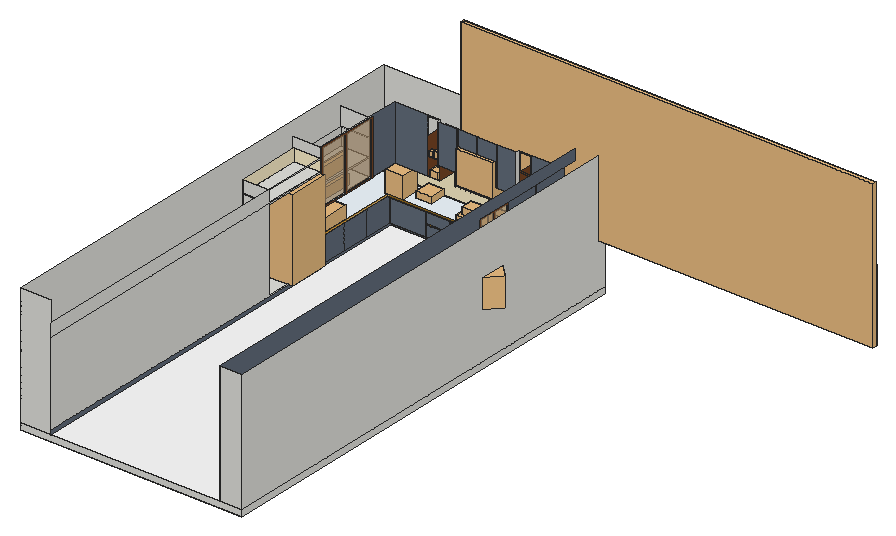
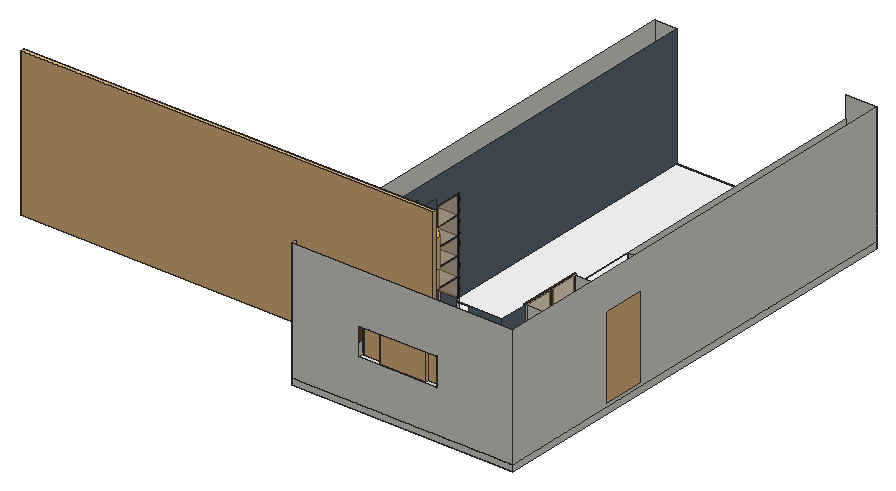
# SketchUp Ruby script. Lengths in inches.
U = 1.inch
M = Sketchup.active_model
def pt(a) = Geom::Point3d.new(a.map { |v| v * U })
def face(e, loops, mat)
  f = e.add_face(loops[0].map { |a| pt(a) })
  loops[1..].each { |l| e.add_face(l.map { |a| pt(a) }).erase! }
  f.material = f.back_material = mat if mat
  f
end
# faces: each face lists its corners as indices into pts; further lists are holes
def faces(e, pts, list, mat = nil) = list.each { |f| face(e, (f[0].is_a?(Array) ? f : [f]).map { |l| l.map { |i| pts[i] } }, mat) }
# xy, xz, yz: faces in a plane at the given z, y or x. An outline is a flat list of corners, or four numbers for a rectangle; further outlines are holes
def ring(l) = l.size == 4 ? [[l[0], l[1]], [l[2], l[1]], [l[2], l[3]], [l[0], l[3]]] : l.each_slice(2).to_a
def flat(e, list, mat, &to3) = list.each { |f| face(e, (f[0].is_a?(Array) ? f : [f]).map { |l| ring(l).map { |u, v| to3.(u, v) } }, mat) }
def xy(e, z, list, mat = nil) = flat(e, list, mat) { |x, y| [x, y, z] }
def xz(e, y, list, mat = nil) = flat(e, list, mat) { |x, z| [x, y, z] }
def yz(e, x, list, mat = nil) = flat(e, list, mat) { |y, z| [x, y, z] }
def lines(e, pts, list) = list.each { |a, b| e.add_line(pt(pts[a]), pt(pts[b])) }
# prism: a flat outline (further loops are holes) pulled along v
def prism(e, loops, v, mat = nil)
  f = face(e, loops, mat); d = Geom::Vector3d.new(v.map { |x| x * U })
  f.pushpull(f.normal.samedirection?(d) ? d.length : -d.length)
end
def box(e, o, s, mat = nil) = prism(e, [[o, [o[0] + s[0], o[1], o[2]], [o[0] + s[0], o[1] + s[1], o[2]], [o[0], o[1] + s[1], o[2]]]], [0, 0, s[2]], mat)
def at(x, y, z, deg = 0) = Geom::Transformation.translation(pt([x, y, z])) * Geom::Transformation.rotation(ORIGIN, Z_AXIS, deg.degrees)
def axes(o, x, y, z) = Geom::Transformation.new([*x, 0, *y, 0, *z, 0, *pt(o).to_a, 1])
def part(name) = M.definitions.add(name)
# library, detail: a bought-in or finely detailed component or shape, given as its bounding box
def library(name, o, s) = part(name).tap { |d| box(d.entities, o, s) }
def detail(e, o, s) = box(e.add_group.entities, o, s)
def put(e, d, t, mat = nil) = e.add_instance(d, t).tap { |i| i.material = mat if mat }
def group(e, t, mat = nil) = e.add_group.tap { |g| g.transformation = t; g.material = mat if mat }.entities
root = M.entities
M.materials.add("Generic").color = [255, 255, 255]
M.materials.add("Material__1").color = [189, 132, 57]
M.materials.add("Material__10").color = [180, 24, 1]
M.materials.add("Material__2").color = [242, 239, 230]
M.materials.add("Material__3").color = [122, 114, 11]
M.materials.add("Picture1").color = [252, 165, 11]
M.materials["Picture1"].alpha = 0.49
M.materials.add("[0093_AliceBlue]").color = [240, 248, 255]
M.materials.add("[0099_LightSteelBlue]").color = [99, 110, 124]
M.materials.add("[Color D01]").color = [255, 242, 204]
M.materials.add("[Color M00]").color = [255, 255, 255]
M.materials.add("[Color M08]").color = [30, 30, 30]
M.materials.add("[Mirror 02]").color = [198, 167, 126]
M.materials["[Mirror 02]"].alpha = 0.66
M.materials.add("[Wood Veneer 01]").color = [120, 70, 37]
M.materials.add("yellow-wall-texture-with-scratches_1249-77").color = [225, 172, 69]
M.materials["yellow-wall-texture-with-scratches_1249-77"].alpha = 0.79
c1 = library("B36CD50SNS_tradeCAD",[0,0,0],[35.84,30.35,69.65])
c2 = library("Oven",[-9.26,-22.59,0.07],[23.42,23.91,23.21])
c3 = library("Component_12",[0,0,0],[17.72,31.5,20.63])
c4 = library("CURA_RiceCooker001_fullGeometry",[-5.98,-7.38,0],[12.22,14.74,12.26])
c5 = library("jars",[-134.79,-4.32,0],[83.43,13.28,34.83])
c6 = library("Floor plant",[-5.56,-16.3125,0.81],[76.88,76.71,92.33])
c7 = library("Group\#314",[-0.26,-0.32,0],[3.72,4.79,9.78])
c8 = library("Group\#29",[55.69,-19.19,40.37],[80.08,80.05,323.81])
c9 = library("Group\#6",[0.46,121.12,-0.1],[106.94,106.94,338.14])
c10 = library("Group\#5",[151.35,137.54,-0.1],[70.51,70.14,256.45])
c11 = library("C_HOB",[0,0,0],[30.71,17.32,2.28])
c12 = library("Group\#33",[70.57,7290.35,1177],[106.36,95.58,107.8])
c13 = library("Group\#46",[141.6875,7219.59,1077.95],[111.05,77.92,100.97])
c14 = library("Group\#32",[73.8125,7223.02,1078.11],[130.55,102.07,69.6])
c15 = library("Group\#18",[51.66,7209.26,1075.25],[220.83,167.48,13.5625])
c16 = library("Group\#45",[99.22,7286.02,1075.87],[101.63,96.21,134.31])
c17 = library("Group\#47",[180.93,7251.18,1124.56],[65.88,104.93,74.66])
c18 = library("vm_v2_031",[-4.73,-4.73,0],[9.46,9.46,3.85])
c19 = library("pot",[774.13,1152.94,114],[93.39,93.39,63.05])
c20 = library("pot (1)",[31.4375,7.2,0.01],[13.32,10.03,8.54])
c21 = library("Kitchen Utensil.",[-24.86,-2.29,-26.5],[81.83,11.85,18.87])
c22 = library("Group\#305",[-29.59,-17.125,-248.78],[31.69,28.84,690.25])
c23 = library("Group1\#1",[6269.2,-3517.56,1634.27],[24.06,1609.34,28.44])
c24 = library("Group2",[6233.88,-3496.88,232.62],[78.05,1568,1448.71])
c25 = library("Group5",[6269.2,-3517.7,1199.35],[24.07,1609.51,427.52])
c26 = library("Group4",[1036.28,1705.4375,-185.71],[3176.52,4429.74,188])
c27 = library("Group3",[6262.98,-3517.7,358.33],[36.34,1611.53,831.81])
c28 = part("Component\#14")
g1 = group(c28.entities,at(-10.68,1.95,4.76),"[Color M00]")
put(g1,c22,axes([23.14,-0.3,14.16],[0,0.01831,0],[-0.00003,0,0.01479],[0.09301,0,0.00001]))
put(g1,c23,axes([140.32,80.99,-2.26],[0,-0.01299,0],[0.03988,0,0],[0,0,0.00972]))
put(g1,c24,axes([140.32,80.99,-2.26],[0,-0.01299,0],[0.03988,0,0],[0,0,0.00972]))
put(g1,c25,axes([140.32,80.99,-2.26],[0,-0.01299,0],[0.03988,0,0],[0,0,0.00972]))
put(g1,c26,axes([453.5,-0.87,-26.375],[-0.10583,0,-0.00001],[-0.00003,0,0.01683],[0,0.02083,0]))
put(g1,c27,axes([140.32,80.99,-2.26],[0,-0.01299,0],[0.03988,0,0],[0,0,0.00972]))
c29 = library("Sliding+Window+Aluminium",[0,0,0],[47.24,2.91,49.21])
c30 = part("KITCHEN WINDOW")
put(c30.entities,c28,axes([5.29,0,-9.32],[0,1.21595,0],[-1,0,0],[0,0,1.95846]),"[Color M00]")
put(c30.entities,c29,axes([2.91,0,0],[0,0.95003,0],[-1,0,0],[0,0,0.57302]))
c31 = library("Untitled (21)",[34.56,5.78,0],[33.51,33.52,23.62])
c32 = library("Group\#261",[-433.81,-170.65,316.14],[99.3,128.23,183.55])
c33 = library("Group\#262",[-328.66,-188.67,316.12],[151.64,146.26,158.64])
c34 = library("Food+jars (1)",[-3.15,-4.1,0],[15.4,16.05,11.47])
c35 = library("Group\#16",[-397.46,82.38,-0.11],[62.88,62.86,260])
c36 = library("Group\#14",[-282.65,82.375,-0.11],[62.85,62.875,260.02])
c37 = library("Group\#15",[222.96,189.98,-0.44],[259.48,39.25,337.49])
c38 = library("Group\#30",[41.52,-158.49,40.25],[95.93,90.14,172.87])
c39 = library("Group\#13",[-504.125,120.57,-0.1],[108.2,108.21,338.13])
c40 = library("Group\#12",[-376.9,120.94,-0.1],[107.79,107.8,326.37])
c41 = library("Group\#11",[-254.81,120.48,-0.6],[108.21,108.21,334.5])
c42 = library("Group\#10",[-133.01,121.19,-0.1],[106.95,106.95,324.89])
c43 = library("Group\#27",[-266.02,-201.27,40.23],[225.02,228.69,89.38])
c44 = library("Group\#28",[-78.56,-74.98,40.25],[131.28,107.59,245.3125])
c45 = library("Group\#31",[-60.55,-181.2,40.41],[105.85,106.35,65.49])
c46 = library("Group\#34",[253.59,42.68,151.97],[53.13,53.13,100.94])
c47 = library("Group\#35",[281.12,-5,151.97],[53.13,53.13,100.92])
c48 = library("Group\#36",[308.75,-52.85,151.97],[53.125,53.13,100.94])
c49 = library("Group\#37",[336.19,-100.38,151.98],[53.13,53.13,100.93])
c50 = library("Group\#38",[363.79,-148.1875,151.98],[53.13,53.13,100.93])
c51 = library("Group\#39",[253.59,42.68,30.7],[53.13,53.13,100.93])
c52 = library("Group\#40",[281.12,-5,30.7],[53.13,53.13,100.91])
c53 = library("Group\#41",[308.75,-52.85,30.7],[53.125,53.13,100.94])
c54 = library("Group\#42",[336.19,-100.38,30.7],[53.13,53.13,100.91])
c55 = library("Group\#43",[363.79,-148.1875,30.7],[53.13,53.13,100.93])
c56 = library("Group\#44",[212.54,-198.04,-0.24],[263.36,352.65,298.47])
c57 = part("KITCHEN+ITEMS+(1) (1)")
put(c57.entities,c35,at(0,0,0))
put(c57.entities,c36,at(0,0,0))
put(c57.entities,c37,at(0,0,0))
put(c57.entities,c38,at(0,0,-41.3))
put(c57.entities,c39,at(0,0,0))
put(c57.entities,c40,at(0,0,0))
put(c57.entities,c41,at(0,0,0))
put(c57.entities,c42,at(0,0,0))
put(c57.entities,c9,at(0,0,0))
put(c57.entities,c10,at(0,0,0))
put(c57.entities,c43,at(0,0,-41.3))
put(c57.entities,c44,at(0,0,-41.3))
put(c57.entities,c45,at(0,0,-41.3))
put(c57.entities,c46,at(0,0,0))
put(c57.entities,c47,at(0,0,0))
put(c57.entities,c48,at(0,0,0))
put(c57.entities,c49,at(0,0,0))
put(c57.entities,c50,at(0,0,0))
put(c57.entities,c51,at(0,0,0))
put(c57.entities,c52,at(0,0,0))
put(c57.entities,c53,at(0,0,0))
put(c57.entities,c54,at(0,0,0))
put(c57.entities,c55,at(0,0,0))
put(c57.entities,c56,at(0,0,0))
put(c57.entities,c8,at(0,0,-41.3))
c58 = library("Group\#260",[0,0,0],[30.82,7.02,10])
c59 = library("PV977NSS_GEProfile",[-17.9375,-27.5625,-0.25],[35.95,27.64,32.08])
c60 = library("Group\#252",[395.59,-144.07,554.28],[103.86,103.86,170.6])
c61 = library("Group\#253",[278.63,-144.07,554.28],[103.86,103.86,170.6])
c62 = library("Group\#254",[163.08,-144.02,554.28],[103.75,103.76,170.6])
c63 = library("Group\#120",[0,0,0],[7.01,7.02,8.25])
c64 = library("Group\#121",[0,0,0],[7,7.02,8.25])
c65 = library("KITCHEN+ITEMS+(3)",[-2.27,-9.02,0],[4.03,10.9,5.45])
xy(root,-6,[[0,0,220,450.125]])
xy(root,0,[[0,0,30,0,30,335,28.4375,335,28.4375,423.125,198,423.125,198,0,220,0,220,450.125,0,450.125]])
xy(root,0,[[30,0,198,0,198,423.125,28.4375,423.125,28.4375,335,30,335]],"Generic")
xy(root,1.01,[[198,271.14,218.5625,296.01]])
xy(root,4,[[28.4375,335,30,363.375],[198,354.34,198.25,354.64],[28.4375,363.375,29.75,363.68],[28.4375,363.68,30,391.75],[198,387.08,198.25,387.38],
  [28.4375,391.75,29.75,392.05],[28.4375,392.05,30,420.125],[28.4375,420.125,30,423.125],[30,420.125,30,423.125,198,423.125,198,420.125,162.3,420.125,162.3,420.375,162,420.375,162,420.125,148.11,420.125,148.11,420.375,147.8125,420.375,147.8125,420.125,138.3,420.125,138.3,420.375,138,420.375,138,420.125,90.3,420.125,90.3,420.375,90,420.375,90,420.125,66.3,420.125,66.3,420.375,66,420.375,66,420.125],[30,423.125,198,444.125]])
xy(root,4.56,[[4.125,270.68,30,334.44]])
xy(root,14.83,[[66.3,420.125,90,420.375],[90.3,420.125,138,420.375]])
xy(root,16,[[66.3,420.125,90,420.375],[90.3,420.125,138,420.375]])
xy(root,16.55,[[198,354.64,198.25,387.08],[198,387.38,198.25,405.02]])
xy(root,17.8,[[198,354.64,198.25,387.08],[198,387.38,198.25,405.02]])
xy(root,17.91,[[198,271.14,218.5625,296.01]])
xy(root,19.16,[[198,271.14,218.5625,296.01]])
xy(root,19.5,[[6.85,342.875,28.23,368.375]])
xy(root,20.5625,[[198,297.58,219,321.38]])
xy(root,23.49,[[90.3,420.125,138,420.375]])
xy(root,24.79,[[90.3,420.125,138,420.375]])
xy(root,28,[[198,354.34,198.25,354.64],[29.75,363.375,30,363.68],[198,387.08,198.25,387.38],[29.75,391.75,30,392.05],[30,418.125,30,420.125,66,420.125,66,420.375,66.3,420.375,66.3,420.125,90,420.125,90,420.375,90.3,420.375,90.3,420.125,138,420.125,138,420.375,138.3,420.375,138.3,420.125,147.8125,420.125,147.8125,420.375,148.11,420.375,148.11,420.125,162,420.125,162,420.375,162.3,420.375,162.3,420.125,198,420.125,198,418.125],
  [30,420.125,30,444.125,198,444.125,198,420.125,162.3,420.125,162.3,420.375,162,420.375,162,420.125,148.11,420.125,148.11,420.375,147.8125,420.375,147.8125,420.125,138.3,420.125,138.3,420.375,138,420.375,138,420.125,90.3,420.125,90.3,420.375,90,420.375,90,420.125,66.3,420.125,66.3,420.375,66,420.375,66,420.125],[30,444.125,198,445.125]])
xy(root,30,[[30,444.125,198,445.125]])
xy(root,30,[[[198,321.9,217,321.9,217,444.125,4.125,444.125,4.125,335,30,335,30,418.125,198,418.125],[6.85,342.875,28.23,368.375]]],"[0093_AliceBlue]")
xy(root,36.5625,[[198,271.14,218.5625,296.01]])
xy(root,37.3125,[[198,271.14,218.5625,296.01]])
xy(root,41.71,[[75.375,444.125,76.375,444.125,76.375,445.125],[75.375,444.125,76.375,445.125,76.375,444.125,153.5625,444.125,153.5625,450.125,75.375,450.125]])
xy(root,45.21,[[198,297.58,219,321.38]])
xy(root,47.25,[[198,297.58,219,321.38]])
xy(root,54,[[198,321.9,198,356.64,198.3,356.64,198.3,356.94,197.6875,356.94,197.6875,408.75,198,408.75,198,426.125,217,426.125,217,321.9],[4.125,335,4.125,444.125,75.375,444.125,75.375,426.125,30,426.125,30,335],[153.5625,426.125,217,444.125]],"[0099_LightSteelBlue]")
xy(root,54.47,[[198,271.14,218.5625,296.01]])
xy(root,54.54,[[154.0625,426.125,165.5625,448.75]],"[Wood Veneer 01]")
xy(root,54.6,[[63.375,426.125,74.78,448.75]],"[Wood Veneer 01]")
xy(root,54.64,[[198,322.54,215.4375,356]])
xy(root,54.89,[[197.6875,357.27,219.8125,407.18]],"[Wood Veneer 01]")
xy(root,54.99,[[0.8125,335.99,30,396.27]])
xy(root,55.47,[[198,271.14,218.5625,296.01]])
xy(root,69.8125,[[75.375,422.75,75.375,450.125,153.5625,450.125,153.5625,422.75,134.32,422.75,134.32,423.05,134.02,423.05,134.02,422.75,114.77,422.75,114.77,423.05,114.47,423.05,114.47,422.75,95.22,422.75,95.22,423.05,94.92,423.05,94.92,422.75]],"[0099_LightSteelBlue]")
xy(root,70.6,[[197.6875,357.27,219.8125,407.18]],"[Wood Veneer 01]")
xy(root,71.24,[[197.6875,356.94,198,391.08],[197.6875,391.08,198,391.38],[197.6875,391.38,198,408.75]])
xy(root,71.51,[[154.0625,426.125,155.1875,448.75],[155.1875,426.125,165.5625,448.75]],"[Wood Veneer 01]")
xy(root,71.53,[[0.8125,335.99,28.4375,396.27]])
xy(root,72.2,[[154.0625,426.125,165.5625,448.75]])
xy(root,72.2,[[63.375,426.125,74.78,448.75]],"[Wood Veneer 01]")
xy(root,72.37,[[198,322.54,215.4375,339.38],[198,339.38,215.4375,339.91],[198,339.91,215.4375,356]])
xy(root,72.53,[[0.8125,335.99,28.4375,396.27]])
xy(root,72.82,[[63.375,426.125,74.78,448.75]])
xy(root,72.84,[[198,322.54,215.4375,356]])
xy(root,72.93,[[198,271.14,218.5625,296.01]])
xy(root,73.62,[[198,271.14,218.5625,296.01]])
xy(root,76.02,[[198,297.58,219,321.38]])
xy(root,85.63,[[4.125,270.68,30,334.44]])
xy(root,86.74,[[4.125,270.68,30,334.44]])
xz(root,0,[[0,-6,220,0],[0,0,30,120],[198,0,220,120]])
xz(root,270.68,[[4.125,4.56,30,85.63],[4.125,86.74,30,98.53]])
xz(root,271.14,[[198,1.01,218.5625,17.91],[198,19.16,218.5625,36.5625],[198,37.3125,218.5625,54.47],[198,55.47,218.5625,72.93],[198,73.62,218.5625,91.77]])
xz(root,296.01,[[198,1.01,218.5625,17.91],[198,19.16,218.5625,36.5625],[198,37.3125,218.5625,54.47],[198,55.47,218.5625,72.93],[198,73.62,218.5625,91.77]])
xz(root,297.58,[[198,20.5625,219,45.21],[198,47.25,219,76.02]])
xz(root,321.38,[[198,20.5625,219,28],[198,28,219,30],[198,30,219,45.21],[198,47.25,219,54],[198,54,219,76.02]])
xz(root,321.9,[[198,30,217,54]])
xz(root,322.54,[[198,54.64,215.4375,72.37],[198,72.84,215.4375,90.38]])
xz(root,334.44,[[4.125,4.56,30,85.63]])
xz(root,334.44,[[4.125,86.74,30,98.53]],"[Color D01]")
xz(root,335,[[28.4375,0,30,4],[4.125,30,30,54]])
xz(root,335.99,[[0.8125,54.99,0.8125,71.53,28.4375,71.53,28.4375,72.53,0.8125,72.53,0.8125,86.1875,30,86.1875,30,54.99],[0.8125,86.1875,0.8125,89.07,28.4375,89.07,28.4375,90.07,0.8125,90.07,0.8125,107.6,30,107.6,30,86.1875]])
xz(root,342.875,[[6.85,19.5,28.23,30]])
xz(root,354.34,[[198,4,198.25,28]])
xz(root,354.64,[[198,4,198.25,16.55],[198,16.55,198.25,17.8],[198,17.8,198.25,28]])
xz(root,356,[[198,54.64,215.4375,72.37],[198,72.84,215.4375,90.38]])
xz(root,356.64,[[198,54,198.3,108.59]])
xz(root,356.94,[[197.6875,54,198.3,54,198.3,108.59,198,108.59,198,71.24,197.6875,71.24]])
xz(root,357.27,[[197.6875,54.89,219.8125,70.6]])
xz(root,363.375,[[29.75,4,30,28]])
xz(root,363.68,[[29.75,4,30,28]])
xz(root,368.375,[[6.85,19.5,28.23,30]])
xz(root,387.08,[[198,4,198.25,16.55],[198,16.55,198.25,17.8],[198,17.8,198.25,28]])
xz(root,387.38,[[198,4,198.25,16.55],[198,16.55,198.25,17.8],[198,17.8,198.25,28]])
xz(root,391.75,[[29.75,4,30,28]])
xz(root,392.05,[[29.75,4,30,28]])
xz(root,396.27,[[0.8125,54.99,30,54.99,30,107.6,0.8125,107.6,0.8125,90.07,28.4375,90.07,28.4375,89.07,0.8125,89.07,0.8125,72.53,28.4375,72.53,28.4375,71.53,0.8125,71.53]])
xz(root,405.02,[[198,16.55,198.25,17.8]])
xz(root,407.18,[[197.6875,54.89,219.8125,70.6]],"[Wood Veneer 01]")
xz(root,408.75,[[197.6875,54,198,71.24]])
xz(root,418.125,[[30,28,198,30]],"Picture1")
xz(root,420.125,[[30,4,66,28],[66.3,4,90,14.83],[90.3,4,138,14.83],[138.3,4,147.8125,28],[148.11,4,162,28],
  [162.3,4,198,28],[66.3,16,90,28],[90.3,16,138,23.49],[90.3,24.79,138,28]],"[0099_LightSteelBlue]")
xz(root,420.375,[[66,4,66.3,28],[90,4,90.3,28],[138,4,138.3,28],[147.8125,4,148.11,28],[162,4,162.3,28]])
xz(root,420.375,[[66.3,14.83,90,16],[90.3,14.83,138,16],[90.3,23.49,138,24.79]],"Picture1")
xz(root,422.75,[[75.375,69.8125,94.92,108.59],[95.22,69.8125,114.47,108.59],[114.77,69.8125,134.02,108.59],[134.32,69.8125,153.5625,108.59]],"[0099_LightSteelBlue]")
xz(root,423.05,[[94.92,69.8125,95.22,108.59],[114.47,69.8125,114.77,108.59],[134.02,69.8125,134.32,108.59]])
xz(root,423.125,[[28.4375,0,198,4]],"[0099_LightSteelBlue]")
xz(root,426.125,[[30,54,62.83,108.59],[166.25,54,198,108.59]],"[0099_LightSteelBlue]")
xz(root,426.125,[[[62.83,54,75.375,108.59],[63.375,54.6,74.78,107.92]],[[153.5625,54,166.25,108.59],[154.0625,90.4,165.5625,108.12],[154.0625,72.2,165.5625,89.71],[154.0625,54.54,165.5625,71.51]],[63.375,72.2,74.78,72.82]],"[Wood Veneer 01]")
xz(root,444.125,[[30,4,198,28],[30,28,198,30]])
xz(root,444.125,[[4.125,30,217,30,217,54,153.5625,54,153.5625,41.71,75.375,41.71,75.375,54,4.125,54]],"[Color D01]")
xz(root,445.125,[[30,28,198,30]])
xz(root,448.75,[[154.0625,54.54,165.5625,71.51],[63.375,54.6,74.78,72.2],[154.0625,72.2,165.5625,89.71],[63.375,72.82,74.78,90.4]],"[Wood Veneer 01]")
xz(root,450.125,[[0,-6,220,0],[[0,0,220,120],[75.375,41.71,153.5625,69.8125]]])
yz(root,0,[[0,-6,450.125,0],[0,0,450.125,120]])
yz(root,0.8125,[[335.99,54.99,396.27,71.53],[335.99,72.53,396.27,89.07]])
yz(root,4.125,[[270.68,4.56,334.44,85.63]])
yz(root,4.125,[[335,30,444.125,54],[270.68,86.74,334.44,98.53]],"[Color D01]")
yz(root,6.85,[[342.875,19.5,368.375,30]])
yz(root,28.23,[[342.875,19.5,368.375,30]])
yz(root,28.4375,[[335.99,71.53,396.27,72.53]])
yz(root,28.4375,[[335,0,423.125,4]],"[0099_LightSteelBlue]")
yz(root,29.75,[[363.375,4,363.68,28],[391.75,4,392.05,28]])
yz(root,30,[[[0,4,335,86.1875],[270.68,4.56,334.44,85.63]],[420.125,4,444.125,28],[444.125,28,445.125,30],[[335,54,397.27,108.59],[335.99,54.99,396.27,107.6]],[[0,86.1875,335,99.09],[270.68,86.74,334.44,98.53]]])
yz(root,30,[[335,28,418.125,30]],"Picture1")
yz(root,30,[[0,0,335,4],[335,4,363.375,28],[363.68,4,391.75,28],[392.05,4,420.125,28],[397.27,54,426.125,108.59]],"[0099_LightSteelBlue]")
yz(root,63.375,[[426.125,54.6,448.75,72.2],[426.125,72.82,448.75,90.4]],"[Wood Veneer 01]")
yz(root,66,[[420.125,4,420.375,28]])
yz(root,66.3,[[420.125,4,420.375,14.83],[420.125,16,420.375,28]])
yz(root,74.78,[[426.125,54.6,448.75,72.2],[426.125,72.82,448.75,90.4]],"[Wood Veneer 01]")
yz(root,75.375,[[444.125,41.71,450.125,54],[422.75,69.8125,426.125,108.59]])
yz(root,75.375,[[426.125,54,450.125,69.8125]],"[Wood Veneer 01]")
yz(root,90,[[420.125,4,420.375,14.83],[420.125,16,420.375,28]])
yz(root,90.3,[[420.125,4,420.375,14.83],[420.125,16,420.375,23.49],[420.125,24.79,420.375,28]])
yz(root,94.92,[[422.75,69.8125,423.05,108.59]])
yz(root,95.22,[[422.75,69.8125,423.05,108.59]])
yz(root,114.47,[[422.75,69.8125,423.05,108.59]])
yz(root,114.77,[[422.75,69.8125,423.05,108.59]])
yz(root,134.02,[[422.75,69.8125,423.05,108.59]])
yz(root,134.32,[[422.75,69.8125,423.05,108.59]])
yz(root,138,[[420.125,4,420.375,14.83],[420.125,16,420.375,23.49],[420.125,24.79,420.375,28]])
yz(root,138.3,[[420.125,4,420.375,28]])
yz(root,147.8125,[[420.125,4,420.375,28]])
yz(root,148.11,[[420.125,4,420.375,28]])
yz(root,153.5625,[[444.125,41.71,450.125,54],[422.75,69.8125,426.125,108.59]])
yz(root,153.5625,[[426.125,54,450.125,69.8125]],"[Wood Veneer 01]")
yz(root,154.0625,[[426.125,54.54,448.75,71.51],[426.125,72.2,448.75,89.71]],"[Wood Veneer 01]")
yz(root,162,[[420.125,4,420.375,28]])
yz(root,162.3,[[420.125,4,420.375,28]])
yz(root,165.5625,[[426.125,54.54,448.75,71.51],[426.125,72.2,448.75,89.71]],"[Wood Veneer 01]")
yz(root,197.6875,[[[356.94,54,408.75,71.24],[357.27,54.89,407.18,70.6]]],"[Wood Veneer 01]")
yz(root,198,[[354.34,4,354.64,28],[387.08,4,387.38,16.55],[420.125,4,444.125,28],[387.08,16.55,387.38,17.8],[387.08,17.8,387.38,28],
  [271.14,17.91,296.01,19.16],[[297.0625,20.04,321.9,45.73],[297.58,20.5625,321.38,45.21]],[444.125,28,445.125,30],[271.14,36.5625,296.01,37.3125],[297.0625,45.73,321.9,46.73],
  [[297.0625,46.73,321.9,76.54],[297.58,47.25,321.38,76.02]],[[321.9,54,356.64,108.59],[322.54,54.64,356,72.37],[322.54,72.84,356,90.38],[322.54,91.04,356,107.95]],[271.14,54.47,296.01,55.47],[391.08,71.24,391.38,108.59],[271.14,72.93,296.01,73.62]])
yz(root,198,[[321.9,28,418.125,30]],"Picture1")
yz(root,198,[[0,0,0,120,444.125,120,444.125,108.59,321.9,108.59,321.9,100.71,297.04,100.71,297.04,100.15,297.0625,92.9375,268.76,92.9375,268.46,0],[297.0625,0,321.9,20.04],[321.9,0,423.125,4],[321.9,4,354.34,28],[354.64,4,387.08,16.55],
  [387.38,4,387.38,16.55,405.02,16.55,405.02,17.8,387.38,17.8,387.38,28,420.125,28,420.125,4],[354.64,17.8,387.08,28],[408.75,54,408.75,71.24,391.38,71.24,391.38,108.59,426.125,108.59,426.125,54],[356.94,71.24,391.08,108.59],[297.0625,76.54,297.0625,92.9375,297.04,100.15,321.9,100.15,321.9,76.54]],"[0099_LightSteelBlue]")
yz(root,198,[[[268.46,0,268.76,92.9375,297.0625,92.9375,297.0625,0],[271.14,1.01,296.01,91.77]]],"[Color M08]")
yz(root,198,[[271.14,1.01,296.01,17.91],[271.14,19.16,296.01,36.5625],[271.14,37.3125,296.01,54.47],[271.14,55.47,296.01,72.93],[271.14,73.62,296.01,91.77]],"[Mirror 02]")
yz(root,198,[[354.64,16.55,387.08,17.8]],"yellow-wall-texture-with-scratches_1249-77")
yz(root,198.25,[[354.34,4,354.64,28],[387.08,4,387.38,28],[354.64,16.55,387.08,17.8]])
yz(root,198.25,[[387.38,16.55,405.02,17.8]],"yellow-wall-texture-with-scratches_1249-77")
yz(root,198.3,[[356.64,54,356.94,108.59]])
yz(root,215.4375,[[322.54,54.64,356,72.37],[322.54,72.84,356,90.38]])
yz(root,217,[[321.9,30,444.125,54]],"[Color D01]")
yz(root,218.5625,[[271.14,1.01,296.01,17.91],[271.14,19.16,296.01,36.5625],[271.14,37.3125,296.01,54.47],[271.14,55.47,296.01,72.93],[271.14,73.62,296.01,91.77]])
yz(root,219,[[297.58,20.5625,321.38,45.21],[297.58,47.25,321.38,76.02]])
yz(root,219.8125,[[357.27,54.89,407.18,70.6]],"[Wood Veneer 01]")
yz(root,220,[[0,-6,450.125,0],[0,0,450.125,120]])
p = [[207.95,274.79,0],[198,296.01,0],[198,298.35,0],[198,298.35,-2.34],[153.53,444.36,53.89],[167.85,444.125,54],
  [153.5625,444.125,54],[153.53,444.125,54],[153.5625,444.125,69.8125]]
lines(root,p,[[0,1],[2,3],[4,5],[6,7],[7,8]])
put(root,c1,axes([34.86,293.64,4.56],[0,1.1386,0],[-1.16,0,0],[0,0,1.16]))
put(root,c2,axes([218.31,312.19,20.46],[0,-0.99882,0],[1,0,0],[0,0,1.06311]))
put(root,c3,axes([7.16,342.79,20.83],[1.19,0,0],[0,0.8122,0],[0,0,1]))
put(root,c4,at(206.73,344.04,30,180))
put(root,c5,axes([217.02,426.57,30],[0.2077,0,0],[0,0.2077,0],[0,0,0.2077]))
put(root,c6,axes([28.27,421.88,29.8125],[0.23,0,0],[0,0.23,0],[0,0,0.23]))
put(root,c7,at(171.86,428.97,30,180))
g2 = group(root,at(172.19,425.85,30))
put(g2,c8,axes([6.11,1.19,-1.42],[0.0352,0,0],[0,0.0352,0],[0,0,0.0352]))
put(g2,c9,axes([-0.02,-4.26,0.03],[0.0352,0,0],[0,0.0352,0],[0,0,0.0352]))
put(g2,c10,axes([-0.02,-4.26,0.03],[0.0352,0,0],[0,0.0352,0],[0,0,0.0352]))
put(root,c11,axes([94.87,420.74,30],[1.308,0,0],[0,1.308,0],[0,0,1.308]))
g3 = group(root,at(200.95,354.48,30))
g4 = group(g3,at(-2.96,-412.37,-61.43),"Material__1")
detail(g4,[10.46,416.25,61.43],[3.24,3.12,3.51])
put(g3,c12,axes([-2.96,-412.37,-61.43],[0.0572,0,0],[0,0.0572,0],[0,0,0.0572]))
put(g3,c13,axes([-2.96,-412.37,-61.43],[0.0572,0,0],[0,0.0572,0],[0,0,0.0572]),"Material__1")
put(g3,c14,axes([-2.96,-412.37,-61.43],[0.0572,0,0],[0,0.0572,0],[0,0,0.0572]),"Material__3")
put(g3,c15,axes([-2.96,-412.37,-61.43],[0.0572,0,0],[0,0.0572,0],[0,0,0.0572]),"Material__2")
put(g3,c16,axes([-2.96,-412.37,-61.43],[0.0572,0,0],[0,0.0572,0],[0,0,0.0572]))
put(g3,c17,axes([-2.96,-412.37,-61.43],[0.0572,0,0],[0,0.0572,0],[0,0,0.0572]),"Material__10")
put(root,c18,axes([58,435.27,30],[1.62,0,0],[0,1.62,0],[0,0,1.62]))
put(root,c19,axes([2.99,285.06,17.98],[0.1218,0,0],[0,0.1218,0],[0,0,0.1218]))
put(root,c20,at(89.34,420.95,32.97))
put(root,c21,axes([215.49,392.78,56.8125],[0,0.51691,0],[-0.66,0,0],[0,0,0.66]))
put(root,c30,at(88.36,448.48,41.71,-90),"[Color D01]")
put(root,c31,axes([156.44,330.09,47.32],[0.70957,-0.70463,0],[0.70463,0.70957,0],[0,0,1.21]))
g5 = group(root,at(197.53,321.9,54),"[Wood Veneer 01]")
xy(g5,0,[[0,0,0.9375,34.74]])
xy(g5,0.64,[[0,0.64,0.47,17.48],[0.47,0.64,0.9375,17.48],[0,18.01,0.47,34.1],[0.47,18.01,0.9375,34.1]])
xy(g5,53.95,[[0,0.64,0.47,17.48],[0.47,0.64,0.9375,17.48],[0,18.01,0.47,34.1],[0.47,18.01,0.9375,34.1]])
xy(g5,54.59,[[0,0,0.9375,34.74]])
xz(g5,0,[[0,0,0.9375,22.54],[0,22.54,0.9375,54.59]])
xz(g5,0.64,[[0,0.64,0.47,53.95],[0.47,0.64,0.9375,53.95]])
xz(g5,17.48,[[0,0.64,0.47,53.95],[0.47,0.64,0.9375,53.95]])
xz(g5,18.01,[[0,0.64,0.47,53.95],[0.47,0.64,0.9375,53.95]])
xz(g5,34.1,[[0,0.64,0.47,53.95],[0.47,0.64,0.9375,53.95]])
xz(g5,34.74,[[0,0,0.9375,54.59]])
yz(g5,0,[[[0,0,34.74,54.59],[0.64,0.64,17.48,53.95],[18.01,0.64,34.1,53.95]]])
yz(g5,0.47,[[0.64,0.64,17.48,53.95],[18.01,0.64,34.1,53.95]],"[Mirror 02]")
yz(g5,0.9375,[[[0,0,34.74,54.59],[0.64,0.64,17.48,53.95],[18.01,0.64,34.1,53.95]]])
g6 = group(root,at(30,335,54),"[Wood Veneer 01]")
yz(g6,0.66,[[0.99,0.99,28.84,53.6],[30.15,0.99,61.27,53.6]],"[Mirror 02]")
g7 = group(g6,at(0,0,0))
xy(g7,0,[[0,0,1.3125,62.27]])
xy(g7,0.99,[[0,0.99,1.3125,28.84],[0,30.15,1.3125,61.27]])
xy(g7,53.6,[[0,0.99,1.3125,28.84],[0,28.84,1.3125,30.15],[0,30.15,1.3125,61.27]])
xy(g7,54.59,[[0,0,1.3125,62.27]])
xz(g7,0,[[0,0,1.3125,32.1875],[0,32.1875,1.3125,54.59]])
xz(g7,0.99,[[0,0.99,1.3125,32.1875],[0,32.1875,1.3125,53.6]])
xz(g7,28.84,[[0,0.99,1.3125,53.6]])
xz(g7,30.15,[[0,0.99,1.3125,53.6]])
xz(g7,61.27,[[0,0.99,1.3125,53.6]])
xz(g7,62.27,[[0,0,1.3125,54.59]])
yz(g7,0,[[[0,0,62.27,54.59],[30.15,0.99,61.27,53.6],[0.99,0.99,28.84,53.6]]])
yz(g7,1.3125,[[[0,0,62.27,54.59],[30.15,0.99,61.27,53.6],[0.99,0.99,28.84,53.6]]])
g8 = group(root,at(164.85,432.27,54.54))
put(g8,c32,axes([-18.22,-7.92,-13.28],[-0.042,0,0],[0,-0.042,0],[0,0,0.042]))
put(g8,c33,axes([-18.22,-7.92,-13.28],[-0.042,0,0],[0,-0.042,0],[0,0,0.042]))
put(root,c34,axes([71.33,432.1,54.6],[-0.5005,0,0],[0,-0.5005,0],[0,0,0.5005]))
put(root,c57,axes([204.57,385.96,54.92],[0,-0.04208,0],[0.03102,0,0],[0,0,0.03102]))
put(root,c58,at(24.85,345.58,54.99,90))
put(root,c59,at(114.77,446.95,61.5))
g9 = group(root,at(164.93,429.98,72.2))
put(g9,c60,axes([5.01,-5.35,-20.59],[-0.03071,0,0],[0,-0.03715,0],[0,0,0.03715]))
put(g9,c61,axes([5.01,-5.35,-20.59],[-0.03071,0,0],[0,-0.03715,0],[0,0,0.03715]))
put(g9,c62,axes([5.01,-5.35,-20.59],[-0.03071,0,0],[0,-0.03715,0],[0,0,0.03715]))
put(root,c5,axes([24.06,390.95,72.53],[0,0.3552,0],[-0.3552,0,0],[0,0,0.3552]))
put(root,c63,axes([69.08,426.125,72.82],[0.71,0,0],[0,0.71,0],[0,0,0.71]))
put(root,c64,axes([64.4375,426.125,72.82],[0.54,0,0],[0,0.54,0],[0,0,0.54]))
put(root,c65,axes([201.03,341.33,72.84],[1.74,0,0],[0,1.74,0],[0,0,1.74]))
